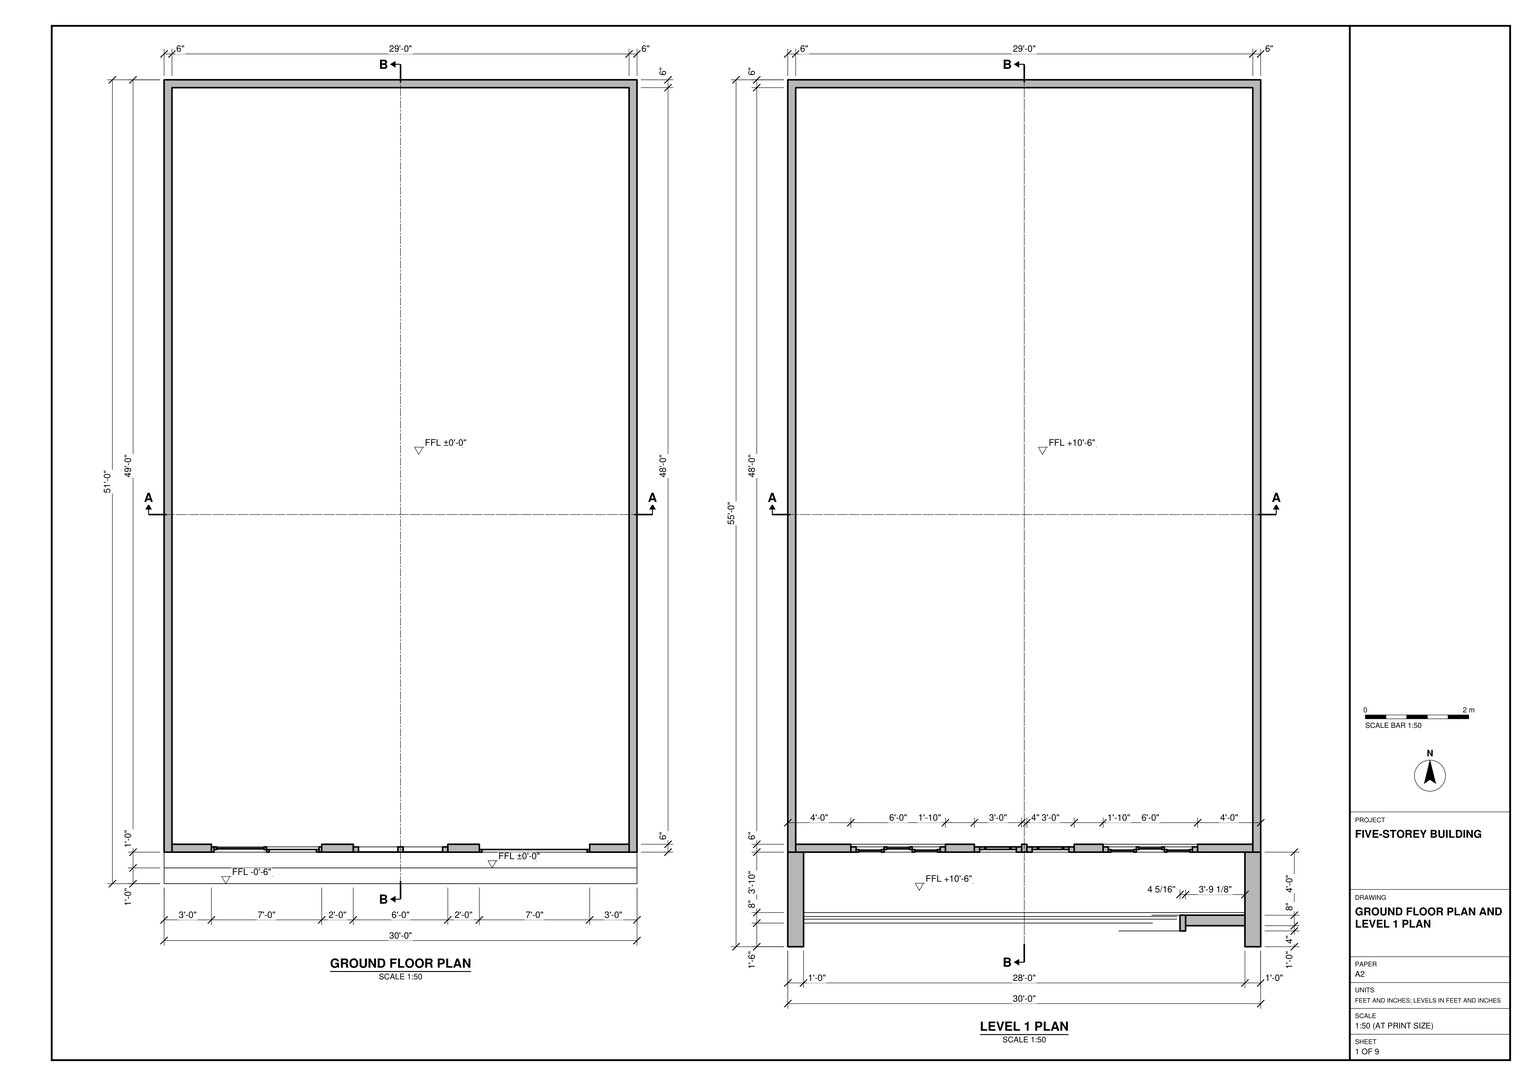
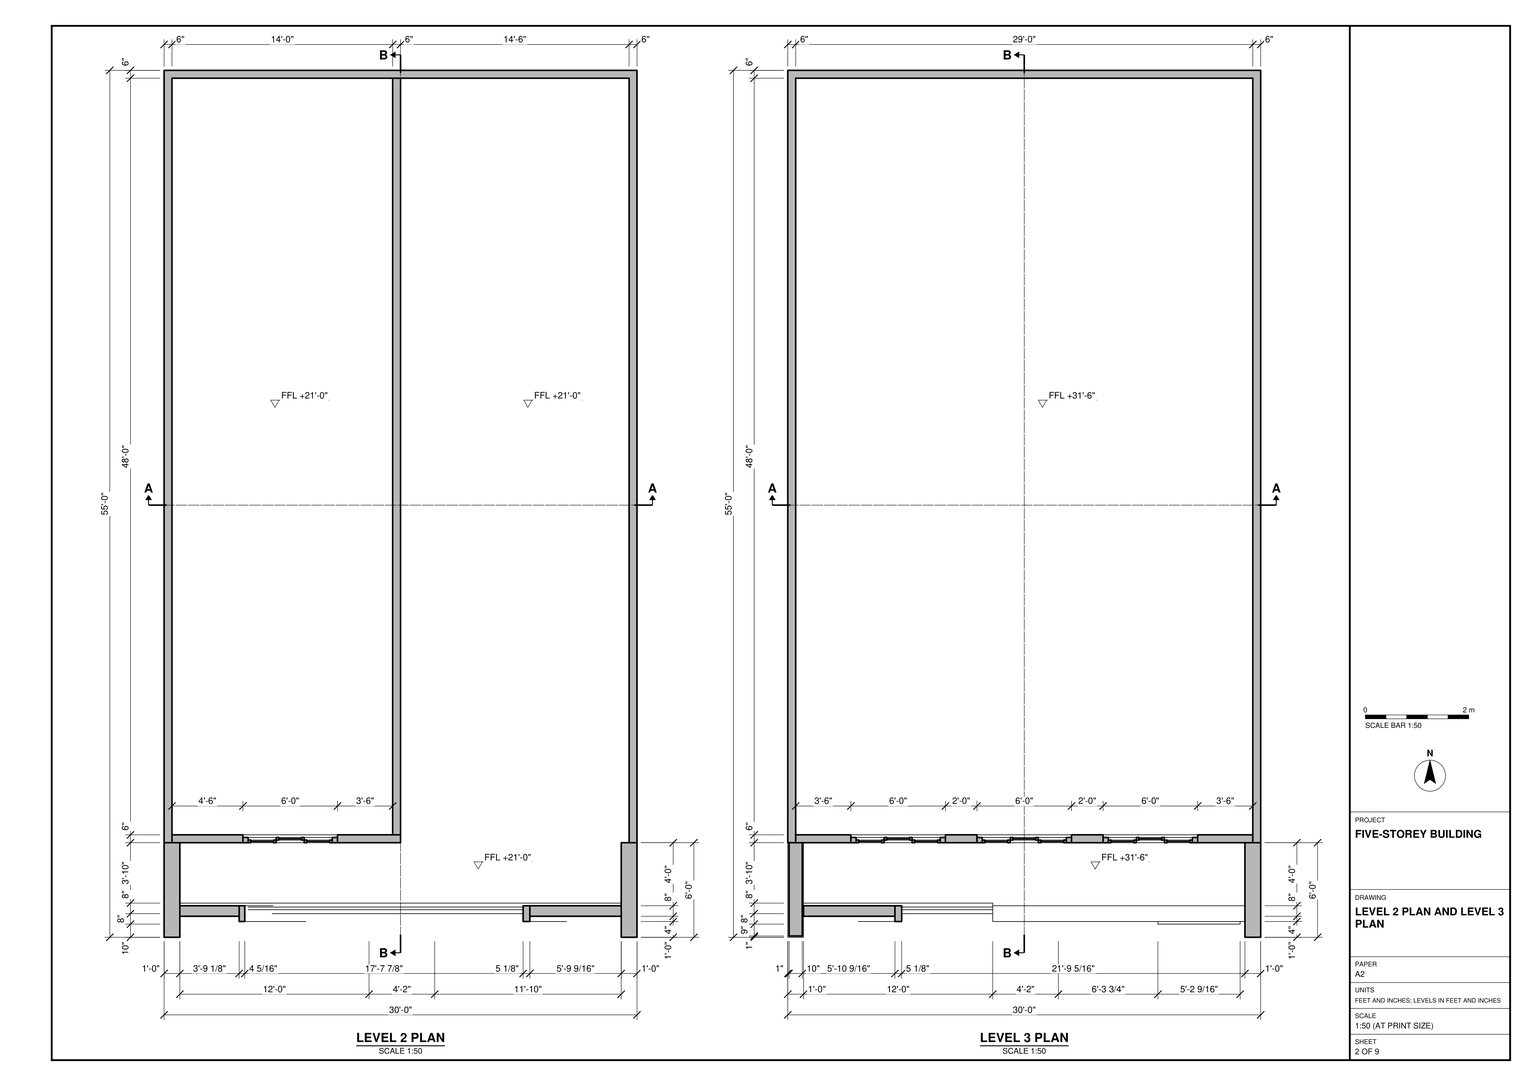
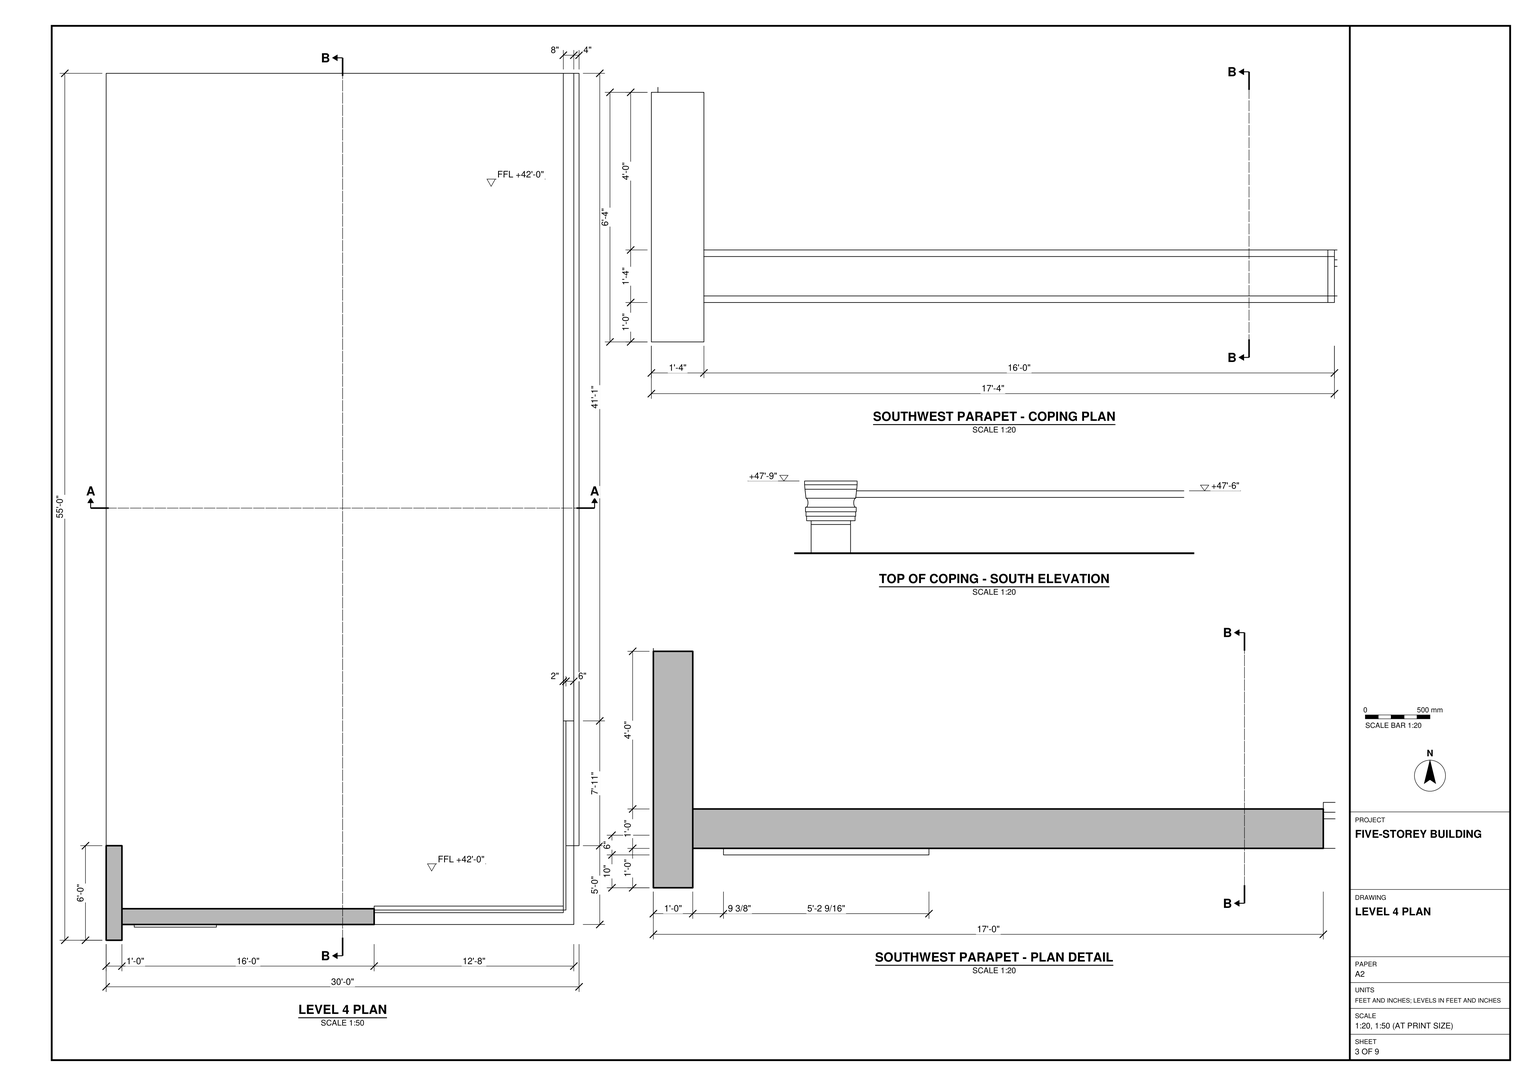
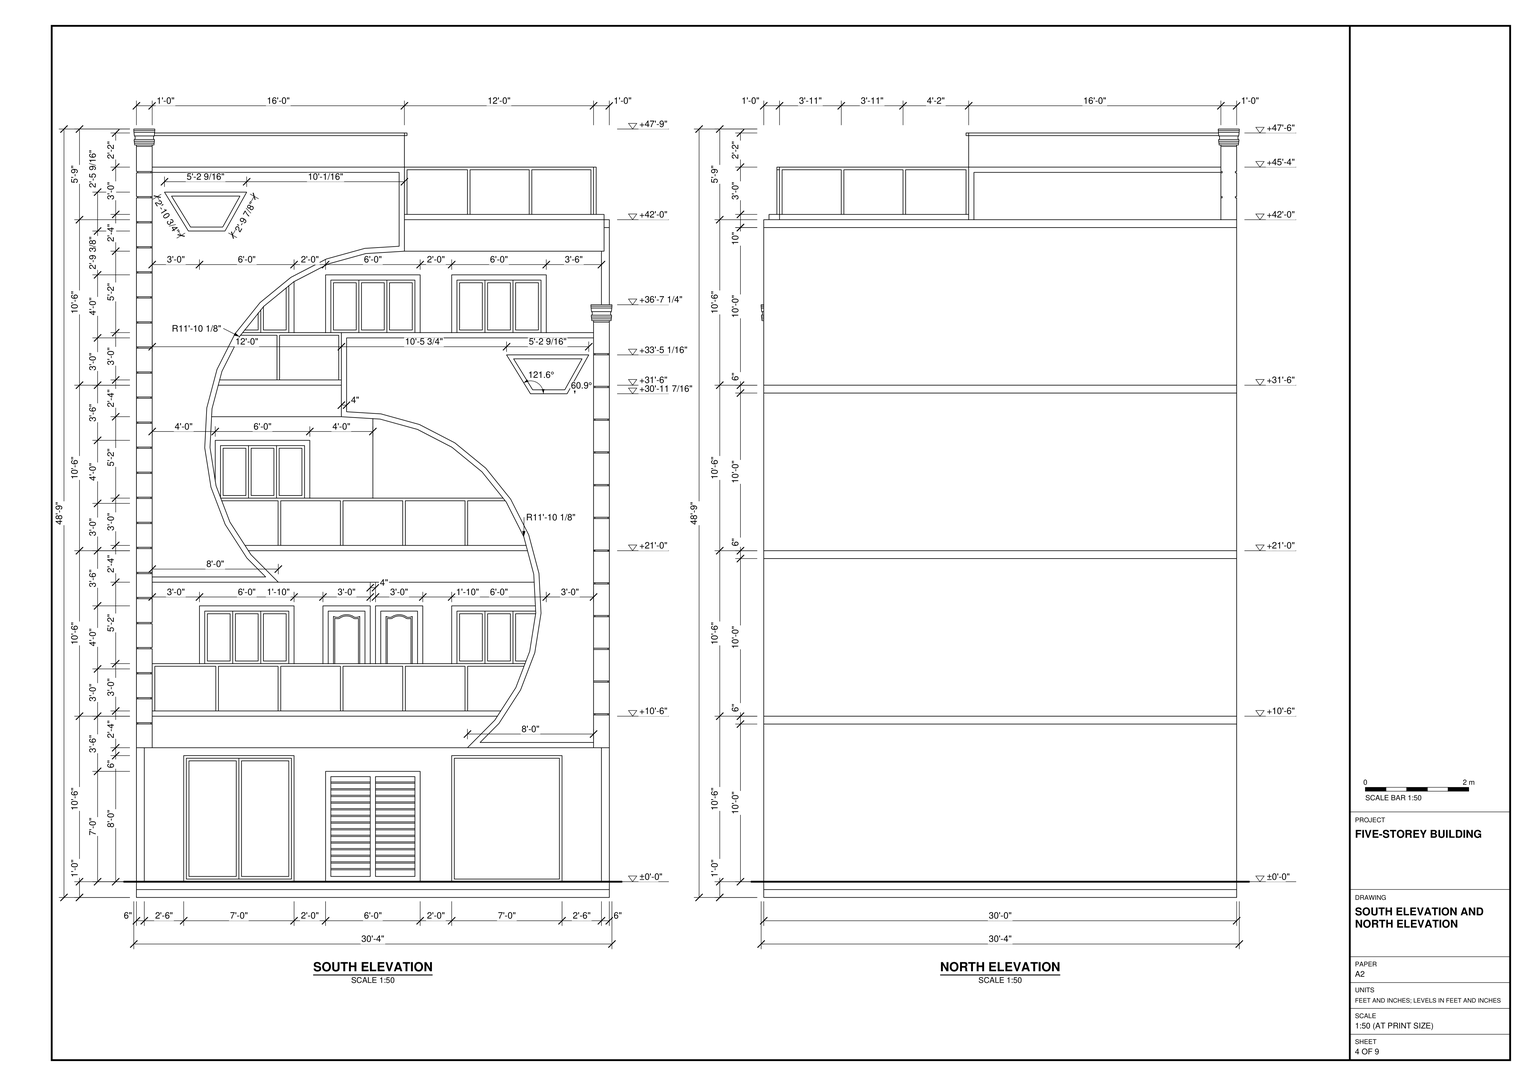
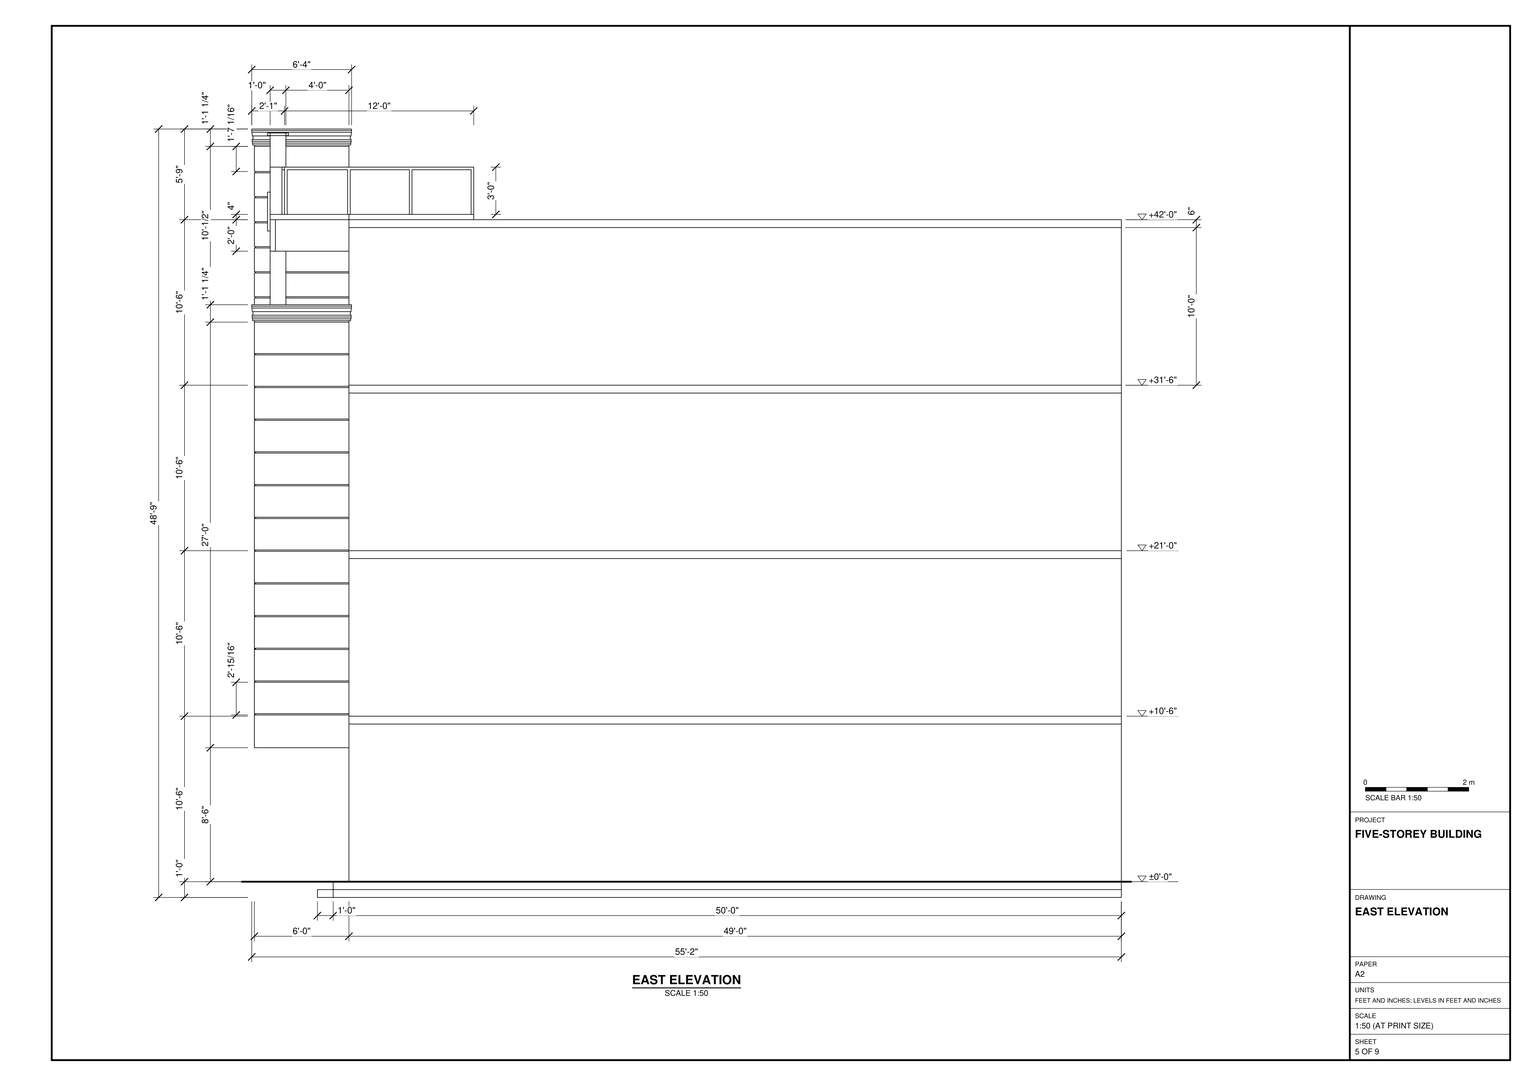
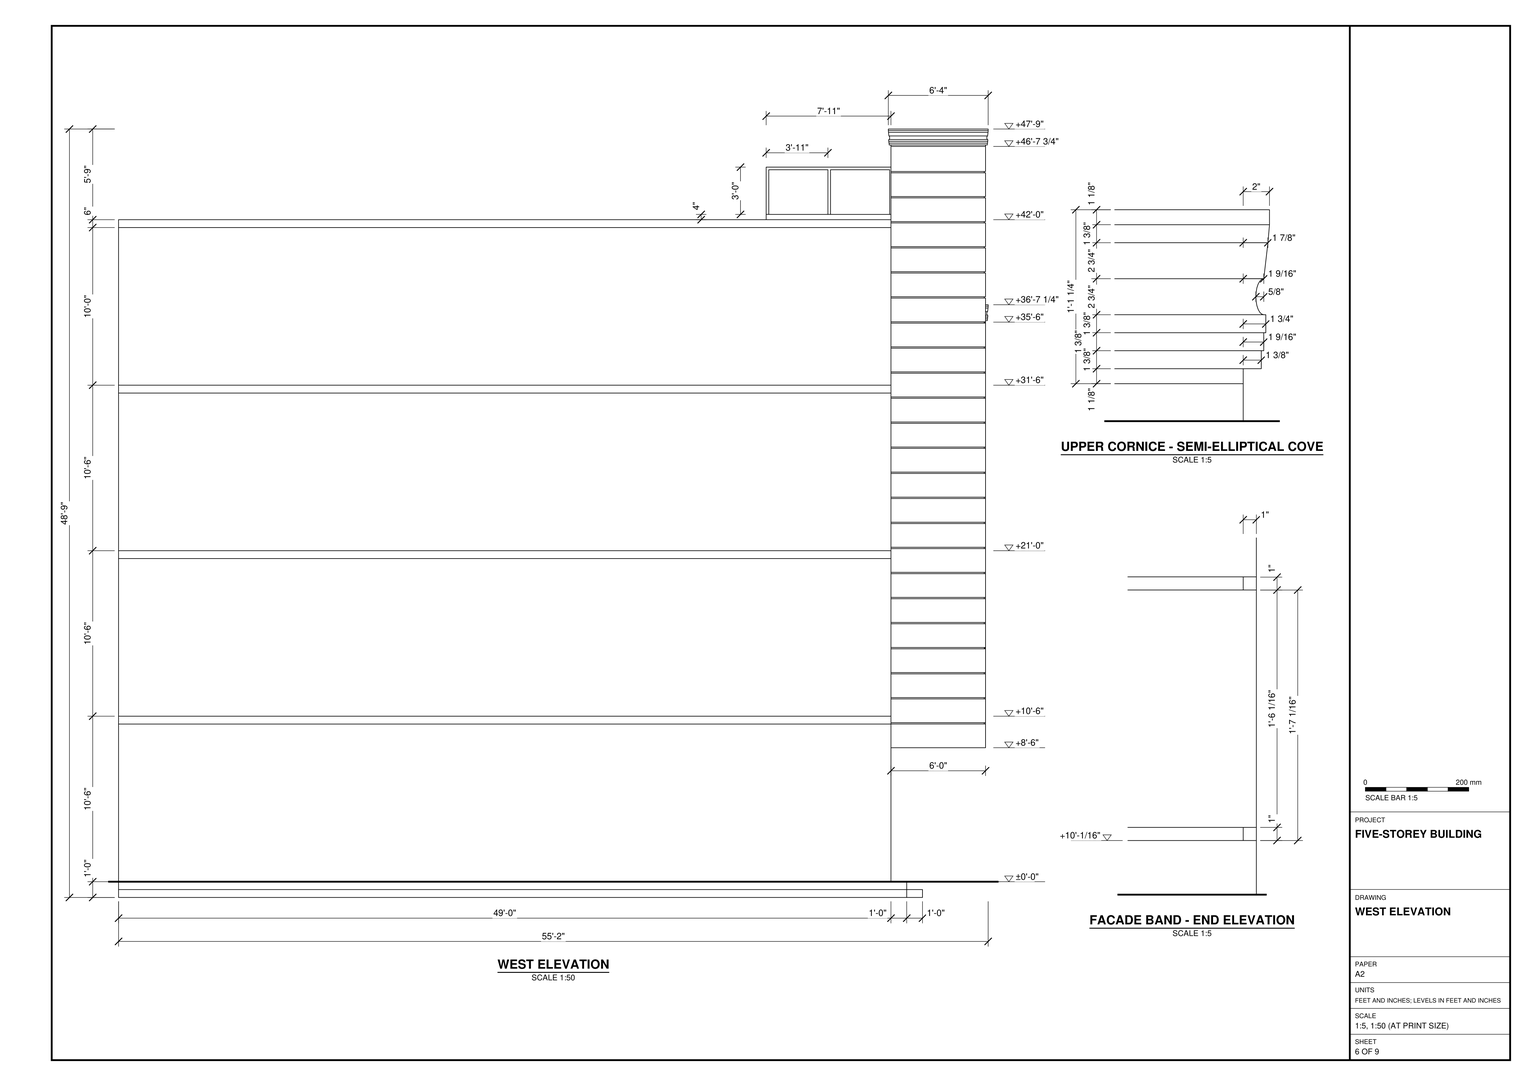
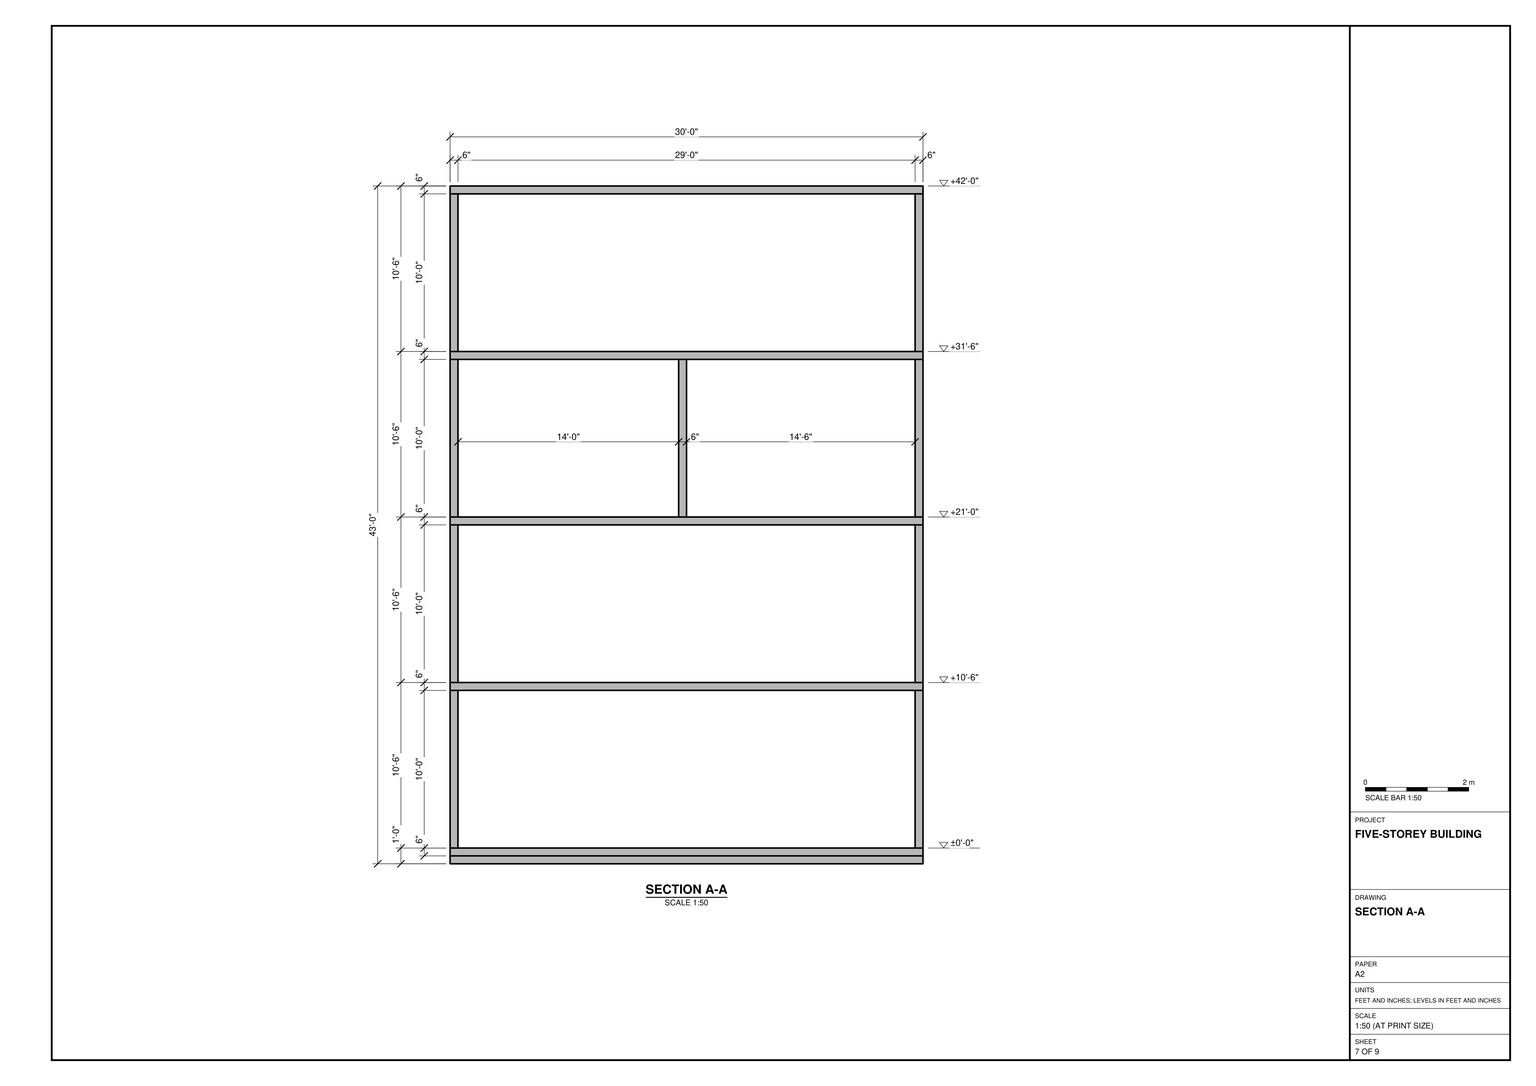
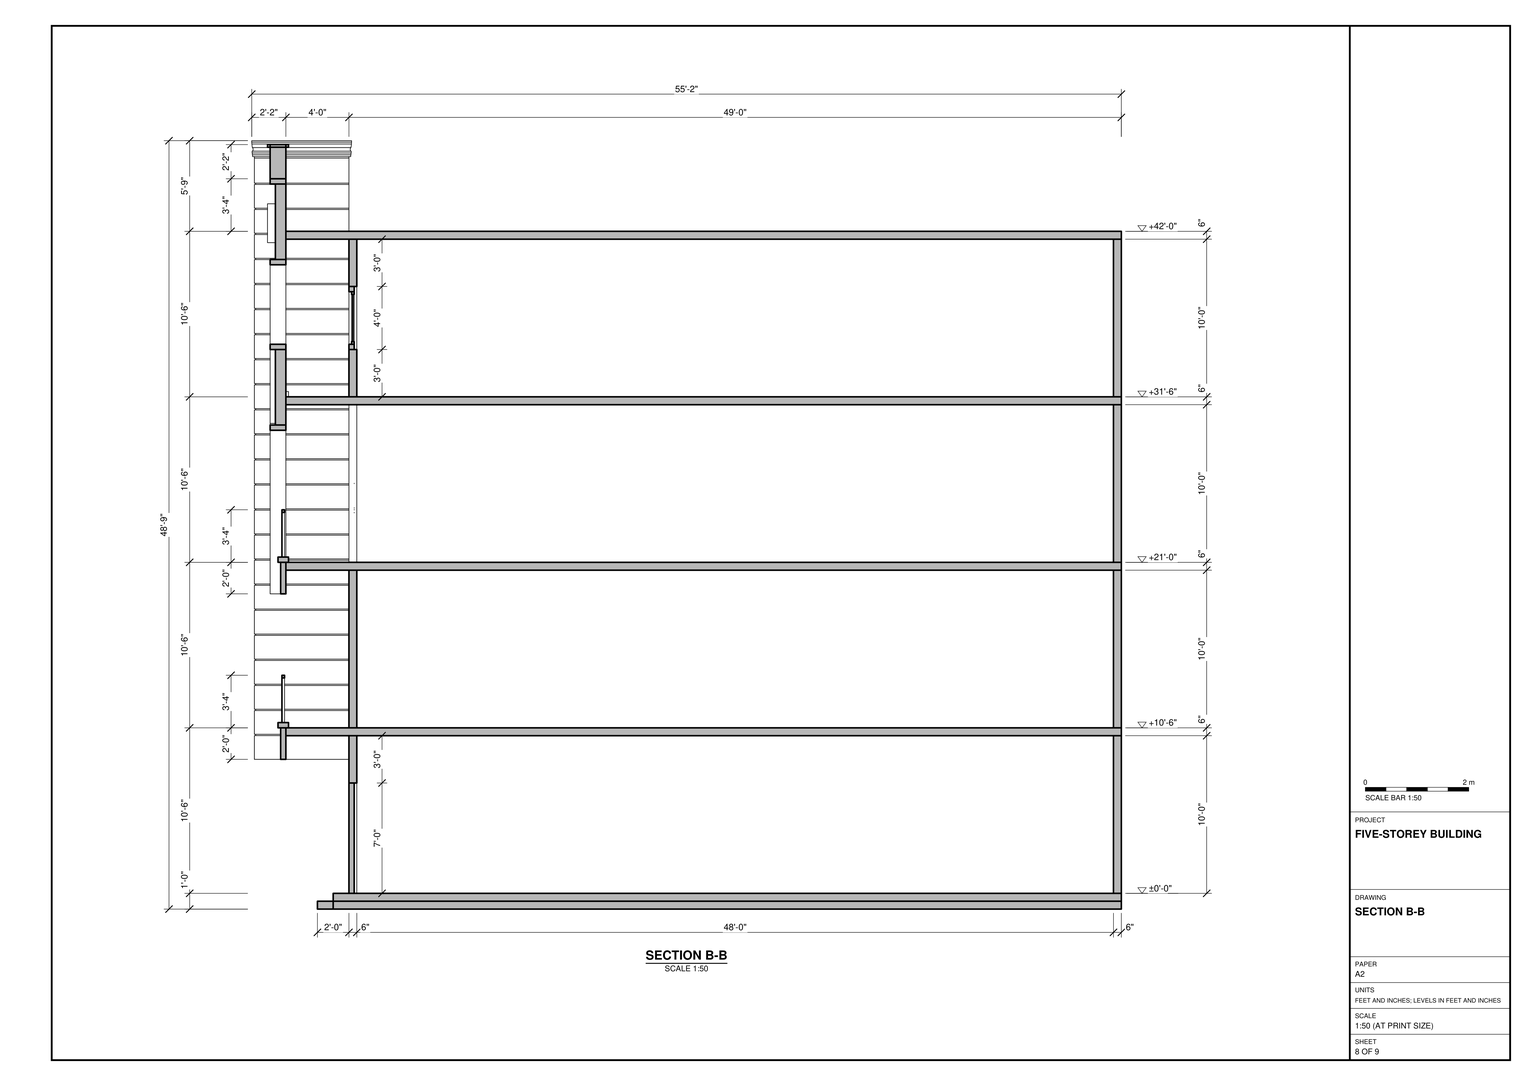
Build the building shown in task_files/diagram_01.pdf in SketchUp. Work in feet and inches. Orient the south frontage along the x axis and the building depth along the y axis. The overall model is 30'-4" wide, 55'-2" deep and 48'-9" high. Set the finished floor levels to ±0'-0", +10'-6", +21'-0", +31'-6" and +42'-0".

Model the floor slabs, perimeter walls and south wall openings from the plans, using the wall thicknesses shown. Include the entrance steps and the door and window units shown in the openings. Keep the ground floor, Level 1 and Level 3 open behind the south wall. On Level 2, run the partition from the rear wall to the south wall of the west bay, leaving the east bay open to the balcony. Follow each level's plan for the projecting balcony slab, side returns and changes in the balcony front rather than copying one balcony unchanged. Model the flat roof at Level 4, including the southwest parapet return and its stepped coping profile.

Make the walls, slabs and roof separate groups or components. Keep each furniture or joinery piece shown separate and use components for repeated parts. Any decor or loose items shown may be represented by suitable library components. Save one SketchUp model as output_files/five_storey_building_with_balconies_and_roof_parapet.skp.

# SketchUp Ruby script. Lengths in inches.
U = 1.inch
M = Sketchup.active_model
def pt(a) = Geom::Point3d.new(a.map { |v| v * U })
def face(e, loops, mat)
  f = e.add_face(loops[0].map { |a| pt(a) })
  loops[1..].each { |l| e.add_face(l.map { |a| pt(a) }).erase! }
  f.material = f.back_material = mat if mat
  f
end
# faces: each face lists its corners as indices into pts; further lists are holes
def faces(e, pts, list, mat = nil) = list.each { |f| face(e, (f[0].is_a?(Array) ? f : [f]).map { |l| l.map { |i| pts[i] } }, mat) }
# xy, xz, yz: faces in a plane at the given z, y or x. An outline is a flat list of corners, or four numbers for a rectangle; further outlines are holes
def ring(l) = l.size == 4 ? [[l[0], l[1]], [l[2], l[1]], [l[2], l[3]], [l[0], l[3]]] : l.each_slice(2).to_a
def flat(e, list, mat, &to3) = list.each { |f| face(e, (f[0].is_a?(Array) ? f : [f]).map { |l| ring(l).map { |u, v| to3.(u, v) } }, mat) }
def xy(e, z, list, mat = nil) = flat(e, list, mat) { |x, y| [x, y, z] }
def xz(e, y, list, mat = nil) = flat(e, list, mat) { |x, z| [x, y, z] }
def yz(e, x, list, mat = nil) = flat(e, list, mat) { |y, z| [x, y, z] }
def lines(e, pts, list) = list.each { |a, b| e.add_line(pt(pts[a]), pt(pts[b])) }
# prism: a flat outline (further loops are holes) pulled along v
def prism(e, loops, v, mat = nil)
  f = face(e, loops, mat); d = Geom::Vector3d.new(v.map { |x| x * U })
  f.pushpull(f.normal.samedirection?(d) ? d.length : -d.length)
end
def box(e, o, s, mat = nil) = prism(e, [[o, [o[0] + s[0], o[1], o[2]], [o[0] + s[0], o[1] + s[1], o[2]], [o[0], o[1] + s[1], o[2]]]], [0, 0, s[2]], mat)
def at(x, y, z, deg = 0) = Geom::Transformation.translation(pt([x, y, z])) * Geom::Transformation.rotation(ORIGIN, Z_AXIS, deg.degrees)
def axes(o, x, y, z) = Geom::Transformation.new([*x, 0, *y, 0, *z, 0, *pt(o).to_a, 1])
def part(name) = M.definitions.add(name)
# library, detail: a bought-in or finely detailed component or shape, given as its bounding box
def library(name, o, s) = part(name).tap { |d| box(d.entities, o, s) }
def detail(e, o, s) = box(e.add_group.entities, o, s)
def put(e, d, t, mat = nil) = e.add_instance(d, t).tap { |i| i.material = mat if mat }
def group(e, t, mat = nil) = e.add_group.tap { |g| g.transformation = t; g.material = mat if mat }.entities
root = M.entities
M.materials.add("[Color C04]").color = [255, 153, 50]
M.materials.add("[Color D01]").color = [255, 242, 204]
M.materials.add("[Color M01]").color = [226, 226, 226]
M.materials.add("[Color M03]").color = [170, 170, 170]
M.materials.add("[Color M04]").color = [142, 142, 142]
M.materials.add("[Mirror 01]").color = [165, 165, 165]
M.materials.add("[Steel Brushed Stainless]").color = [183, 187, 190]
M.materials.add("[Translucent Glass Blue]").color = [100, 149, 237]
M.materials["[Translucent Glass Blue]"].alpha = 0.5
M.materials.add("[Wood Bamboo]").color = [177, 105, 43]
M.materials.add("[Wood Floor Parquet]").color = [145, 89, 39]
c1 = part("Group\#18")
xy(c1.entities,120,[[0,0,6,0,6,582,354,582,354,0,360,0,360,588,0,588]])
xz(c1.entities,0,[[0,0,6,120],[354,0,360,120]])
xz(c1.entities,582,[[6,0,354,120]])
xz(c1.entities,588,[[0,0,360,120]])
yz(c1.entities,0,[[0,0,588,120]])
yz(c1.entities,6,[[0,0,582,120]])
yz(c1.entities,354,[[0,0,582,120]])
yz(c1.entities,360,[[0,0,588,120]])
c2 = part("Group\#11")
prism(c2.entities,[[[50.43,0,0],[48.43,0,0],[48.43,0,34],[2,0,34],[2,0,0],[0,0,0],[0,0,36],[336,0,36],[336,0,0],[334,0,0],[334,0,34],[287.57,0,34],[287.57,0,0],[285.57,0,0],[285.57,0,34],[240.14,0,34],[240.14,0,0],[238.14,0,0],[238.14,0,34],[192.71,0,34],[192.71,0,0],[190.71,0,0],[190.71,0,34],[145.29,0,34],[145.29,0,0],[143.29,0,0],[143.29,0,34],[97.86,0,34],[97.86,0,0],[95.86,0,0],[95.86,0,34],[50.43,0,34]]],[0,-2,0],"[Steel Brushed Stainless]")
c3 = library("Group\#14",[0,-12,0],[12,72,324])
c4 = part("Group\#5")
xy(c4.entities,0,[[0,0,2,2],[48.43,0,50.43,2],[95.86,0,97.86,2],[143.29,0,145.29,2]],"[Steel Brushed Stainless]")
xy(c4.entities,34,[[2,0,48.43,2],[50.43,0,95.86,2],[97.86,0,143.29,2]],"[Steel Brushed Stainless]")
xy(c4.entities,36,[[0,0,145.29,2]],"[Steel Brushed Stainless]")
xz(c4.entities,0,[[0,0,2,0,2,34,48.43,34,48.43,0,50.43,0,50.43,34,95.86,34,95.86,0,97.86,0,97.86,34,143.29,34,143.29,0,145.29,0,145.29,36,0,36]],"[Steel Brushed Stainless]")
xz(c4.entities,0,[[2,0,48.43,34],[50.43,0,95.86,34],[97.86,0,143.29,34]],"[Translucent Glass Blue]")
xz(c4.entities,2,[[0,0,0,36,145.29,36,145.29,0,143.29,0,143.29,34,97.86,34,97.86,0,95.86,0,95.86,34,50.43,34,50.43,0,48.43,0,48.43,34,2,34,2,0]],"[Steel Brushed Stainless]")
yz(c4.entities,0,[[0,0,2,36]],"[Steel Brushed Stainless]")
yz(c4.entities,2,[[0,0,2,34]],"[Steel Brushed Stainless]")
yz(c4.entities,48.43,[[0,0,2,34]],"[Steel Brushed Stainless]")
yz(c4.entities,50.43,[[0,0,2,34]],"[Steel Brushed Stainless]")
yz(c4.entities,95.86,[[0,0,2,34]],"[Steel Brushed Stainless]")
yz(c4.entities,97.86,[[0,0,2,34]],"[Steel Brushed Stainless]")
yz(c4.entities,143.29,[[0,0,2,34]],"[Steel Brushed Stainless]")
yz(c4.entities,145.29,[[0,0,2,34],[0,34,2,36]],"[Steel Brushed Stainless]")
c5 = library("Group\#8",[-2,-2,0],[197.6875,16,342])
c6 = library("Group\#9",[0,0,-0.5],[16,76,5.8])
c7 = part("Group\#22")
prism(c7.entities,[[[21.33,0,0],[0,0,0],[0,0,40],[21.33,0,40]],[[19.33,0,38],[2,0,38],[2,0,2],[19.33,0,2]]],[0,-2,0])
g1 = group(c7.entities,at(2,-1,2))
xz(g1,0,[[0,0,17.33,36]],"[Mirror 01]")
c8 = part("Group\#24")
put(c8.entities,c7,at(25.33,4,4))
put(c8.entities,c7,at(4,2,4))
g2 = group(c8.entities,at(0,0,0))
prism(g2,[[[72,4,0],[0,4,0],[0,4,48],[72,4,48]],[[4,4,44],[4,4,4],[68,4,4],[68,4,44]]],[0,-4,0])
put(c8.entities,c7,at(46.67,2,4))
c9 = library("Group\#27",[0,0,0],[36,4,84])
c10 = library("Group\#35",[0,0,0],[36,4,84])
c11 = library("Group\#13",[0,0,0.1875],[12,72,457.75])
c12 = library("Group\#33",[0,-4,0],[72,4,84])
c13 = part("Group\#38")
xy(c13.entities,0,[[18.2,-6,46.07,0]])
xy(c13.entities,3,[[19.875,-6,44.3125,-2]])
xy(c13.entities,26.59,[[5.37,-6,57.46,-2]])
xy(c13.entities,29.59,[[0,-6,62.5625,0]])
xz(c13.entities,-6,[[[18.2,0,46.07,0,62.5625,29.59,0,29.59],[19.875,3,5.37,26.59,57.46,26.59,44.3125,3]]],"[Color M01]")
xz(c13.entities,-2,[[19.875,3,44.3125,3,57.46,26.59,5.37,26.59]],"[Color M03]")
xz(c13.entities,0,[[[18.2,0,0,29.59,62.5625,29.59,46.07,0],[19.875,3,44.3125,3,57.46,26.59,5.37,26.59]]])
p = [[0,0,29.59],[18.2,0,0],[18.2,-6,0],[0,-6,29.59],[46.07,0,0],[62.5625,0,29.59],
  [62.5625,-6,29.59],[46.07,-6,0],[19.875,-2,3],[5.37,-2,26.59],[5.37,-6,26.59],[19.875,-6,3],
  [57.46,-2,26.59],[44.3125,-2,3],[44.3125,-6,3],[57.46,-6,26.59],[19.875,0,3],[5.37,0,26.59],
  [44.3125,0,3],[57.46,0,26.59]]
faces(c13.entities,p,[[0,1,2,3],[4,5,6,7],[8,9,10,11],[12,13,14,15]])
lines(c13.entities,p,[[16,8],[17,9],[18,13],[19,12]])
xy(root,438,[[350,2,362,74]])
g3 = group(root,at(2,62,0))
xy(g3,0,[[0,-12,360,0],[0,0,360,600]])
xy(g3,6,[[0,-12,360,0],[0,0,360,600]])
xy(g3,12,[[0,0,360,600]])
xz(g3,-12,[[0,0,360,6]])
xz(g3,0,[[0,0,360,6],[0,6,360,12]])
xz(g3,600,[[0,0,360,6],[0,6,360,12]])
yz(g3,0,[[-12,0,0,6],[0,0,600,6],[0,6,600,12]])
yz(g3,360,[[-12,0,0,6],[0,0,600,6],[0,6,600,12]])
put(root,c1,at(2,74,12),"[Color D01]")
g4 = group(root,at(2,38,132),"[Color M01]")
prism(g4,[[[360,624,0],[360,36,0],[348,36,0],[348,-12,0],[12,-12,0],[12,36,0],[0,36,0],[0,624,0]]],[0,0,6])
g5 = group(root,at(2,22,114),"[Color M01]")
xy(g5,0,[[12,0,348,4]],"[Color M04]")
xy(g5,24,[[12,-2,348,0],[12,0,348,4],[12,4,348,6]])
xy(g5,28,[[12,-2,348,6]])
xz(g5,-2,[[12,24,348,28]])
xz(g5,0,[[12,0,348,24]],"[Color M04]")
xz(g5,4,[[12,0,348,24]])
xz(g5,6,[[12,24,348,28]])
yz(g5,12,[[0,0,4,24],[-2,24,6,28]])
yz(g5,348,[[0,0,4,24],[-2,24,6,28]])
g6 = group(root,at(14,23,142))
xz(g6,0,[[0,0,336,36]],"[Translucent Glass Blue]")
put(g6,c2,at(0,2,0))
put(root,c3,at(350,14,114),"[Color M01]")
put(root,c1,at(2,74,138),"[Color M01]")
g7 = group(root,at(2,38,258),"[Color M01]")
prism(g7,[[[360,624,0],[360,36,0],[348,36,0],[348,-12,0],[12,-12,0],[12,36,0],[0,36,0],[0,624,0]]],[0,0,6])
put(root,c1,at(2,74,264),"[Color D01]")
g8 = group(root,at(2,38,384))
xy(g8,0,[[12,-12,12,36,0,36,0,624,360,624,360,36,348,36,348,-12]],"[Color C04]")
xy(g8,6,[[12,-12,348,-12,348,36,360,36,360,624,0,624,0,36,12,36]])
xz(g8,-12,[[12,0,348,6]])
xz(g8,36,[[0,0,12,6],[348,0,360,6]])
xz(g8,624,[[0,0,360,6]])
yz(g8,0,[[36,0,624,6]])
yz(g8,12,[[-12,0,36,6]])
yz(g8,348,[[-12,0,36,6]])
yz(g8,360,[[36,0,624,6]])
g9 = group(root,at(2,74,390),"[Color D01]")
xy(g9,120,[[0,0,6,0,6,582,354,582,354,0,360,0,360,588,0,588]])
xz(g9,0,[[0,0,6,120],[354,0,360,120]])
xz(g9,582,[[6,0,354,120]])
xz(g9,588,[[0,0,360,120]])
yz(g9,0,[[0,0,588,120]])
yz(g9,6,[[0,0,582,120]])
yz(g9,354,[[0,0,582,120]])
yz(g9,360,[[0,0,588,120]])
g10 = group(root,at(2,38,510))
xy(g10,0,[[12,-12,12,36,0,36,0,624,360,624,360,36,348,36,348,-12]])
xy(g10,6,[[12,-12,348,-12,348,624,0,624,0,36,12,36],[348,36,356,131],[356,36,360,624],[348,131,356,624]])
xy(g10,10,[[348,36,356,131]])
xz(g10,-12,[[12,0,348,6]])
xz(g10,36,[[0,0,12,6],[348,0,360,6],[348,6,356,10]])
xz(g10,131,[[348,6,356,10]])
xz(g10,624,[[0,0,360,6]])
yz(g10,0,[[36,0,624,6]])
yz(g10,12,[[-12,0,36,6]])
yz(g10,348,[[-12,0,36,6],[36,6,131,10]])
yz(g10,356,[[36,6,131,10]])
yz(g10,360,[[36,0,624,6]])
g11 = group(root,at(2,22,240),"[Color M01]")
xy(g11,0,[[12,0,348,4]],"[Color M04]")
xy(g11,24,[[12,-2,348,0],[12,0,348,4],[12,4,348,6]])
xy(g11,28,[[12,-2,348,6]])
xz(g11,-2,[[12,24,348,28]])
xz(g11,0,[[12,0,348,24]],"[Color M04]")
xz(g11,4,[[12,0,348,24]])
xz(g11,6,[[12,24,348,28]])
yz(g11,12,[[0,0,4,24],[-2,24,6,28]])
yz(g11,348,[[0,0,4,24],[-2,24,6,28]])
g12 = group(root,at(14,23,268),"[Translucent Glass Blue]")
xz(g12,0,[[0,0,336,36]],"[Translucent Glass Blue]")
put(g12,c2,at(0,2,0))
g13 = group(root,at(2,22,366),"[Color M01]")
xy(g13,0,[[12,0,156,4]],"[Color M04]")
xy(g13,24,[[12,-2,156,0],[12,0,156,4],[12,4,156,6]])
xy(g13,28,[[12,-2,156,6]])
xz(g13,-2,[[12,24,156,28]])
xz(g13,0,[[12,0,156,24]],"[Color M04]")
xz(g13,4,[[12,0,156,24]])
xz(g13,6,[[12,24,156,28]])
yz(g13,12,[[0,0,4,24],[-2,24,6,28]])
yz(g13,156,[[0,0,4,24],[-2,24,6,28]])
put(root,c4,axes([14,23,394],[0.99115,0,0],[0,1,0],[0,0,1]))
g14 = group(root,at(194,22,492))
xy(g14,0,[[12,-4,12,4,156,4,156,52,164,52,164,-4]],"[Color M04]")
xy(g14,24,[[12,-8,164,-4],[12,-4,12,4,156,4,156,52,164,52,164,-4],[12,4,156,6]])
xy(g14,28,[[12,-8,164,-8,164,52,156,52,156,6,12,6]])
xz(g14,-8,[[12,24,164,28]])
xz(g14,-4,[[12,0,164,24]],"[Color M04]")
xz(g14,4,[[12,0,156,24]])
xz(g14,6,[[12,24,156,28]])
xz(g14,52,[[156,0,164,24],[156,24,164,28]])
yz(g14,12,[[-4,0,4,24],[-8,24,6,28]])
yz(g14,156,[[4,0,52,24],[6,24,52,28]])
yz(g14,164,[[-8,24,52,28]])
yz(g14,164,[[-4,0,52,24]],"[Color M04]")
put(root,c4,axes([206,23,520],[0.99115,0,0],[0,1,0],[0,0,1]))
g15 = group(root,at(158,22,114),"[Color M01]")
xy(g15,0,[[96,-8,192,4]])
xy(g15,4,[[105.61,-8,192,-4],[105.61,-4,192,4]])
xy(g15,312,[[4,-8,192,-4],[4,-4,192,4]])
xy(g15,316,[[0,-8,192,4]])
xz(g15,-8,[[96,0,192,0,192,4,105.61,4,119.94,18.45,136.42,43.97,147.27,72.35,152.01,102.35,150.44,132.69,142.64,162.05,128.93,189.16,109.91,212.85,86.41,232.1,59.43,246.07,30.15,254.16,4,255.76,4,312,192,312,192,316,0,316,0,252,29.49,250.19,57.96,242.32,84.2,228.74,107.06,210.02,125.55,186.99,138.88,160.62,146.47,132.07,147.99,102.57,143.38,73.39,132.83,45.79,116.81,20.97]])
xz(g15,-4,[[105.61,4,192,4,192,312,4,312,4,255.76,30.15,254.16,59.43,246.07,86.41,232.1,109.91,212.85,128.93,189.16,142.64,162.05,150.44,132.69,152.01,102.35,147.27,72.35,136.42,43.97,119.94,18.45]],"[Wood Floor Parquet]")
xz(g15,4,[[96,0,116.81,20.97,132.83,45.79,143.38,73.39,147.99,102.57,146.47,132.07,138.88,160.62,125.55,186.99,107.06,210.02,84.2,228.74,57.96,242.32,29.49,250.19,0,252,0,316,192,316,192,312,4,312,4,255.76,30.15,254.16,59.43,246.07,86.41,232.1,109.91,212.85,128.93,189.16,142.64,162.05,150.44,132.69,152.01,102.35,147.27,72.35,136.42,43.97,119.94,18.45,105.61,4,192,4,192,0],[105.61,4,119.94,18.45,136.42,43.97,147.27,72.35,152.01,102.35,150.44,132.69,142.64,162.05,128.93,189.16,109.91,212.85,86.41,232.1,59.43,246.07,30.15,254.16,4,255.76,4,312,192,312,192,4]])
yz(g15,0,[[-8,252,4,316]])
yz(g15,4,[[-8,255.76,-4,312],[-4,255.76,4,312]])
yz(g15,192,[[-8,0,4,4],[-4,4,4,312],[-8,312,4,316]])
p = [[116.81,-8,20.97],[116.81,4,20.97],[96,4,0],[96,-8,0],[105.61,-8,4],[105.61,-4,4],
  [119.94,-4,18.45],[119.94,-8,18.45],[105.61,4,4],[119.94,4,18.45],[136.42,-4,43.97],[136.42,-8,43.97],
  [136.42,4,43.97],[132.83,-8,45.79],[132.83,4,45.79],[147.27,-4,72.35],[147.27,-8,72.35],[147.27,4,72.35],
  [143.38,-8,73.39],[143.38,4,73.39],[152.01,-4,102.35],[152.01,-8,102.35],[152.01,4,102.35],[147.99,-8,102.57],
  [147.99,4,102.57],[150.44,-4,132.69],[150.44,-8,132.69],[150.44,4,132.69],[146.47,-8,132.07],[146.47,4,132.07],
  [138.88,-8,160.62],[138.88,4,160.62],[142.64,-4,162.05],[142.64,-8,162.05],[142.64,4,162.05],[125.55,-8,186.99],
  [125.55,4,186.99],[128.93,-4,189.16],[128.93,-8,189.16],[128.93,4,189.16],[107.06,-8,210.02],[107.06,4,210.02],
  [109.91,-4,212.85],[109.91,-8,212.85],[109.91,4,212.85],[84.2,-8,228.74],[84.2,4,228.74],[86.41,-4,232.1],
  [86.41,-8,232.1],[86.41,4,232.1],[57.96,-8,242.32],[57.96,4,242.32],[59.43,-4,246.07],[59.43,-8,246.07],
  [59.43,4,246.07],[29.49,-8,250.19],[29.49,4,250.19],[30.15,-4,254.16],[30.15,-8,254.16],[30.15,4,254.16],
  [0,-8,252],[0,4,252],[4,-4,255.76],[4,-8,255.76],[4,4,255.76],[192,0,316],
  [195.6875,0,316]]
faces(g15,p,[[0,1,2,3],[4,5,6,7],[5,8,9,6],[7,6,10,11],[6,9,12,10],[13,14,1,0],[11,10,15,16],[10,12,17,15],
  [18,19,14,13],[16,15,20,21],[15,17,22,20],[23,24,19,18],[21,20,25,26],[20,22,27,25],[28,29,24,23],[30,31,29,28],
  [26,25,32,33],[25,27,34,32],[35,36,31,30],[33,32,37,38],[32,34,39,37],[40,41,36,35],[38,37,42,43],[37,39,44,42],
  [45,46,41,40],[43,42,47,48],[42,44,49,47],[50,51,46,45],[48,47,52,53],[47,49,54,52],[55,56,51,50],[53,52,57,58],
  [52,54,59,57],[60,61,56,55],[58,57,62,63],[57,59,64,62]])
lines(g15,p,[[65,66]])
put(root,c5,at(206,26,240,180),"[Color M01]")
put(root,c6,axes([348,0,439.14],[1,0,0],[0,1,0],[0,0,2.2836]))
put(root,c4,axes([352,25,520],[0,0.99115,0],[-1,0,0],[0,0,1]))
g16 = group(root,at(8,74,138),"[Color D01]")
prism(g16,[[[348,6,0],[212,6,0],[212,6,84],[176,6,84],[176,6,0],[172,6,0],[172,6,84],[136,6,84],[136,6,0],[0,6,0],[0,6,120],[348,6,120]],[[306,6,84],[234,6,84],[234,6,36],[306,6,36]],[[114,6,36],[114,6,84],[42,6,84],[42,6,36]]],[0,-6,0])
g17 = group(root,at(8,74,264),"[Color D01]")
xy(g17,0,[[0,0,174,6],[168,6,174,582]])
xy(g17,36,[[54,0,126,6]])
xy(g17,84,[[54,0,126,6]])
xy(g17,120,[[0,0,174,6],[168,6,174,582]])
xz(g17,0,[[[0,0,174,120],[54,36,126,84]]])
xz(g17,6,[[[0,0,168,120],[54,36,126,84]],[168,0,174,120]])
xz(g17,582,[[168,0,174,120]])
yz(g17,0,[[0,0,6,120]])
yz(g17,54,[[0,36,6,84]])
yz(g17,126,[[0,36,6,84]])
yz(g17,168,[[6,0,582,120]])
yz(g17,174,[[0,0,6,120],[6,0,582,120]])
g18 = group(root,at(8,74,390),"[Color D01]")
prism(g18,[[[348,6,0],[0,6,0],[0,6,120],[348,6,120]],[[114,6,84],[42,6,84],[42,6,36],[114,6,36]],[[234,6,36],[306,6,36],[306,6,84],[234,6,84]],[[138,6,84],[138,6,36],[210,6,36],[210,6,84]]],[0,-6,0])
put(root,c8,at(62,74,300),"[Steel Brushed Stainless]")
put(root,c6,axes([0,0,572.89],[1,0,0],[0,1,0],[0,0,2.2836]))
put(root,c8,at(50,74,174),"[Steel Brushed Stainless]")
put(root,c8,at(242,74,174),"[Steel Brushed Stainless]")
put(root,c9,at(144,74,138),"[Wood Bamboo]")
put(root,c10,at(184,74,138),"[Wood Bamboo]")
put(root,c8,at(50,74,426),"[Steel Brushed Stainless]")
put(root,c8,at(146,74,426),"[Steel Brushed Stainless]")
put(root,c8,at(242,74,426),"[Steel Brushed Stainless]")
put(root,c11,at(2,2,113.8125),"[Color M01]")
g19 = group(root,at(8,74,12),"[Color D01]")
prism(g19,[[[348,6,0],[318,6,0],[318,6,96],[234,6,96],[234,6,0],[210,6,0],[210,6,84],[138,6,84],[138,6,0],[114,6,0],[114,6,96],[30,6,96],[30,6,0],[0,6,0],[0,6,120],[348,6,120]]],[0,-6,0])
g20 = group(g19,at(30,0,0),"[Steel Brushed Stainless]")
g21 = group(g20,at(0,0,0))
xy(g21,2,[[42,0,82,2]])
xy(g21,4,[[44,0,80,2]])
xy(g21,92,[[44,0,80,2]])
xy(g21,94,[[42,0,82,2]])
xz(g21,0,[[[42,2,82,94],[44,4,80,92]]])
xz(g21,2,[[[42,2,82,94],[44,4,80,92]]])
xz(g21,2,[[44,4,80,92]],"[Translucent Glass Blue]")
yz(g21,42,[[0,2,2,94]])
yz(g21,44,[[0,4,2,92]])
yz(g21,80,[[0,4,2,92]])
yz(g21,82,[[0,2,2,94]])
g22 = group(g21,at(4,3,4),"[Translucent Glass Blue]")
xz(g22,0,[[0,0,36,88]])
g23 = group(g21,at(0,0,0))
xy(g23,0,[[0,0,84,4]])
xy(g23,2,[[2,0,42,2],[42,0,82,4],[2,2,42,4]])
xy(g23,4,[[4,2,40,4]])
xy(g23,92,[[4,2,40,4]])
xy(g23,94,[[2,0,42,2],[42,0,82,4],[2,2,42,4]])
xy(g23,96,[[0,0,84,4]])
xz(g23,0,[[[0,0,84,96],[2,2,82,94]]])
xz(g23,2,[[[2,2,42,94],[4,4,40,92]]])
xz(g23,4,[[[0,0,84,96],[2,2,82,94]],[[2,2,42,94],[4,4,40,92]]])
yz(g23,0,[[0,0,4,96]])
yz(g23,2,[[0,2,2,94],[2,2,4,94]])
yz(g23,4,[[2,4,4,92]])
yz(g23,40,[[2,4,4,92]])
yz(g23,42,[[2,2,4,94]])
yz(g23,82,[[0,2,4,94]])
yz(g23,84,[[0,0,4,96]])
g24 = group(g19,at(234,0,0))
g25 = group(g24,at(0,2,0),"[Steel Brushed Stainless]")
xy(g25,0,[[0,-2,84,0]])
xy(g25,2,[[2,-2,82,0]])
xy(g25,94,[[2,-2,82,0]])
xy(g25,96,[[0,-2,84,0]])
xz(g25,-2,[[[0,0,84,96],[2,2,82,94]]])
xz(g25,0,[[[0,0,84,96],[2,2,82,94]]])
xz(g25,0,[[2,2,82,94]],"[Translucent Glass Blue]")
yz(g25,0,[[-2,0,0,96]])
yz(g25,2,[[-2,2,0,94]])
yz(g25,82,[[-2,2,0,94]])
yz(g25,84,[[-2,0,0,96]])
put(g19,c12,at(138,4,0),"[Steel Brushed Stainless]")
put(root,c13,at(23.36,18,507.37),"[Color M01]")
put(root,c13,at(283.77,18,383.47),"[Color M01]")
